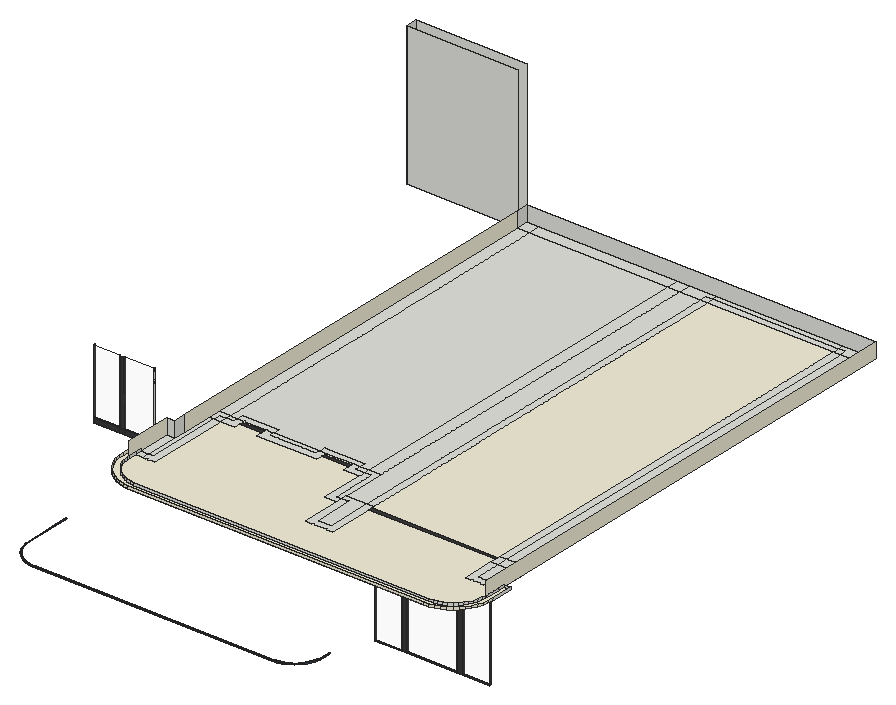
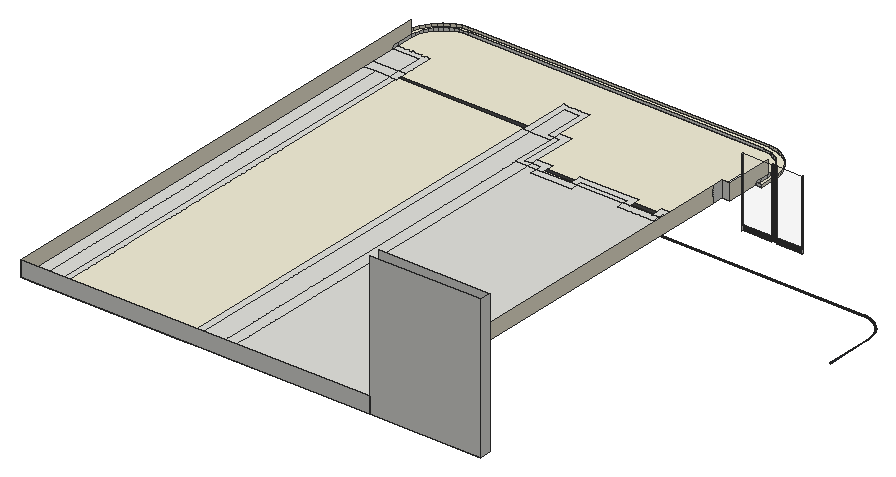
# SketchUp Ruby script. Lengths in inches.
U = 1.inch
M = Sketchup.active_model
def pt(a) = Geom::Point3d.new(a.map { |v| v * U })
def face(e, loops, mat)
  f = e.add_face(loops[0].map { |a| pt(a) })
  loops[1..].each { |l| e.add_face(l.map { |a| pt(a) }).erase! }
  f.material = f.back_material = mat if mat
  f
end
# faces: each face lists its corners as indices into pts; further lists are holes
def faces(e, pts, list, mat = nil) = list.each { |f| face(e, (f[0].is_a?(Array) ? f : [f]).map { |l| l.map { |i| pts[i] } }, mat) }
# xy, xz, yz: faces in a plane at the given z, y or x. An outline is a flat list of corners, or four numbers for a rectangle; further outlines are holes
def ring(l) = l.size == 4 ? [[l[0], l[1]], [l[2], l[1]], [l[2], l[3]], [l[0], l[3]]] : l.each_slice(2).to_a
def flat(e, list, mat, &to3) = list.each { |f| face(e, (f[0].is_a?(Array) ? f : [f]).map { |l| ring(l).map { |u, v| to3.(u, v) } }, mat) }
def xy(e, z, list, mat = nil) = flat(e, list, mat) { |x, y| [x, y, z] }
def xz(e, y, list, mat = nil) = flat(e, list, mat) { |x, z| [x, y, z] }
def yz(e, x, list, mat = nil) = flat(e, list, mat) { |y, z| [x, y, z] }
def lines(e, pts, list) = list.each { |a, b| e.add_line(pt(pts[a]), pt(pts[b])) }
# prism: a flat outline (further loops are holes) pulled along v
def prism(e, loops, v, mat = nil)
  f = face(e, loops, mat); d = Geom::Vector3d.new(v.map { |x| x * U })
  f.pushpull(f.normal.samedirection?(d) ? d.length : -d.length)
end
def box(e, o, s, mat = nil) = prism(e, [[o, [o[0] + s[0], o[1], o[2]], [o[0] + s[0], o[1] + s[1], o[2]], [o[0], o[1] + s[1], o[2]]]], [0, 0, s[2]], mat)
def at(x, y, z, deg = 0) = Geom::Transformation.translation(pt([x, y, z])) * Geom::Transformation.rotation(ORIGIN, Z_AXIS, deg.degrees)
def axes(o, x, y, z) = Geom::Transformation.new([*x, 0, *y, 0, *z, 0, *pt(o).to_a, 1])
def part(name) = M.definitions.add(name)
# library, detail: a bought-in or finely detailed component or shape, given as its bounding box
def library(name, o, s) = part(name).tap { |d| box(d.entities, o, s) }
def detail(e, o, s) = box(e.add_group.entities, o, s)
def put(e, d, t, mat = nil) = e.add_instance(d, t).tap { |i| i.material = mat if mat }
def group(e, t, mat = nil) = e.add_group.tap { |g| g.transformation = t; g.material = mat if mat }.entities
root = M.entities
M.materials.add("0360 AP 9644 Monsoon Midnight-N").color = [56, 67, 95]
M.materials.add("0905 AP 7844 MILD YELLOW").color = [242, 237, 215]
M.materials.add("Glass Clear 001").color = [246, 246, 246]
M.materials["Glass Clear 001"].alpha = 0.1
M.materials.add("[Color M07]").color = [58, 58, 58]
xy(root,164.31,[[267.15,94.4375,287.73,95.4375],[291.07,94.4375,329.62,95.4375],[333.85,94.4375,354.31,95.4375]],"[Color M07]")
xy(root,168,[[57,32.3125,54.18,32.5,51.4,33.05,48.72,33.96,46.1875,35.21,43.84,36.78,41.71,38.65,39.84,40.77,38.27,43.125,37.02,45.66,36.11,48.34,35.56,51.11,35.375,53.9375,35.375,89.9375,35.75,89.9375,35.75,53.9375,35.94,51.16,36.48,48.4375,37.37,45.81,38.6,43.3125,40.14,41,41.98,38.91,44.07,37.08,46.375,35.54,48.87,34.31,51.5,33.41,54.23,32.87,57,32.69,238.5625,32.69,241.34,32.87,244.0625,33.41,246.69,34.31,249.1875,35.54,251.5,37.08,253.59,38.91,255.42,41,256.96,43.3125,258.19,45.81,259.09,48.4375,259.63,51.16,259.81,53.9375,259.81,60.0625,260.1875,60.0625,260.1875,53.9375,260,51.11,259.45,48.34,258.54,45.66,257.29,43.125,255.72,40.77,253.85,38.65,251.73,36.78,249.375,35.21,246.84,33.96,244.16,33.05,241.39,32.5,238.5625,32.3125]])
xy(root,168,[[[57,32.18,54.16,32.36,51.37,32.92,48.67,33.83,46.12,35.09,43.75,36.68,41.61,38.55,39.74,40.69,38.16,43.06,36.9,45.61,35.98,48.31,35.43,51.1,35.24,53.9375,35.24,90.07,35.89,90.07,35.89,53.9375,36.07,51.18,36.61,48.47,37.49,45.86,38.72,43.38,40.25,41.08,42.07,39.01,44.15,37.1875,46.44,35.65,48.92,34.43,51.54,33.54,54.24,33,57,32.82,238.5625,32.82,241.32,33,244.03,33.54,246.64,34.43,249.12,35.65,251.42,37.1875,253.49,39.01,255.3125,41.08,256.85,43.38,258.07,45.86,258.96,48.47,259.5,51.18,259.68,53.9375,259.68,60.2,260.32,60.2,260.32,53.9375,260.14,51.1,259.58,48.31,258.67,45.61,257.41,43.06,255.82,40.69,253.95,38.55,251.81,36.68,249.44,35.09,246.89,33.83,244.19,32.92,241.4,32.36,238.5625,32.18],[57,32.3125,238.5625,32.3125,241.39,32.5,244.16,33.05,246.84,33.96,249.375,35.21,251.73,36.78,253.85,38.65,255.72,40.77,257.29,43.125,258.54,45.66,259.45,48.34,260,51.11,260.1875,53.9375,260.1875,60.0625,259.81,60.0625,259.81,53.9375,259.63,51.16,259.09,48.4375,258.19,45.81,256.96,43.3125,255.42,41,253.59,38.91,251.5,37.08,249.1875,35.54,246.69,34.31,244.0625,33.41,241.34,32.87,238.5625,32.69,57,32.69,54.23,32.87,51.5,33.41,48.87,34.31,46.375,35.54,44.07,37.08,41.98,38.91,40.14,41,38.6,43.3125,37.37,45.81,36.48,48.4375,35.94,51.16,35.75,53.9375,35.75,89.9375,35.375,89.9375,35.375,53.9375,35.56,51.11,36.11,48.34,37.02,45.66,38.27,43.125,39.84,40.77,41.71,38.65,43.84,36.78,46.1875,35.21,48.72,33.96,51.4,33.05,54.18,32.5]]],"0360 AP 9644 Monsoon Midnight-N")
xy(root,168.1875,[[[57,32.18,54.16,32.36,51.37,32.92,48.67,33.83,46.12,35.09,43.75,36.68,41.61,38.55,39.74,40.69,38.16,43.06,36.9,45.61,35.98,48.31,35.43,51.1,35.24,53.9375,35.24,90.07,35.89,90.07,35.89,53.9375,36.07,51.18,36.61,48.47,37.49,45.86,38.72,43.38,40.25,41.08,42.07,39.01,44.15,37.1875,46.44,35.65,48.92,34.43,51.54,33.54,54.24,33,57,32.82,238.5625,32.82,241.32,33,244.03,33.54,246.64,34.43,249.12,35.65,251.42,37.1875,253.49,39.01,255.3125,41.08,256.85,43.38,258.07,45.86,258.96,48.47,259.5,51.18,259.68,53.9375,259.68,60.2,260.32,60.2,260.32,53.9375,260.14,51.1,259.58,48.31,258.67,45.61,257.41,43.06,255.82,40.69,253.95,38.55,251.81,36.68,249.44,35.09,246.89,33.83,244.19,32.92,241.4,32.36,238.5625,32.18],[57,32.3125,238.5625,32.3125,241.39,32.5,244.16,33.05,246.84,33.96,249.375,35.21,251.73,36.78,253.85,38.65,255.72,40.77,257.29,43.125,258.54,45.66,259.45,48.34,260,51.11,260.1875,53.9375,260.1875,60.0625,259.81,60.0625,259.81,53.9375,259.63,51.16,259.09,48.4375,258.19,45.81,256.96,43.3125,255.42,41,253.59,38.91,251.5,37.08,249.1875,35.54,246.69,34.31,244.0625,33.41,241.34,32.87,238.5625,32.69,57,32.69,54.23,32.87,51.5,33.41,48.87,34.31,46.375,35.54,44.07,37.08,41.98,38.91,40.14,41,38.6,43.3125,37.37,45.81,36.48,48.4375,35.94,51.16,35.75,53.9375,35.75,89.9375,35.375,89.9375,35.375,53.9375,35.56,51.11,36.11,48.34,37.02,45.66,38.27,43.125,39.84,40.77,41.71,38.65,43.84,36.78,46.1875,35.21,48.72,33.96,51.4,33.05,54.18,32.5]],[57,32.3125,54.18,32.5,51.4,33.05,48.72,33.96,46.1875,35.21,43.84,36.78,41.71,38.65,39.84,40.77,38.27,43.125,37.02,45.66,36.11,48.34,35.56,51.11,35.375,53.9375,35.375,89.9375,35.75,89.9375,35.75,53.9375,35.94,51.16,36.48,48.4375,37.37,45.81,38.6,43.3125,40.14,41,41.98,38.91,44.07,37.08,46.375,35.54,48.87,34.31,51.5,33.41,54.23,32.87,57,32.69,238.5625,32.69,241.34,32.87,244.0625,33.41,246.69,34.31,249.1875,35.54,251.5,37.08,253.59,38.91,255.42,41,256.96,43.3125,258.19,45.81,259.09,48.4375,259.63,51.16,259.81,53.9375,259.81,60.0625,260.1875,60.0625,260.1875,53.9375,260,51.11,259.45,48.34,258.54,45.66,257.29,43.125,255.72,40.77,253.85,38.65,251.73,36.78,249.375,35.21,246.84,33.96,244.16,33.05,241.39,32.5,238.5625,32.3125]],"0360 AP 9644 Monsoon Midnight-N")
xy(root,168.3125,[[[57,32.18,238.5625,32.18,241.4,32.36,244.19,32.92,246.89,33.83,249.44,35.09,251.81,36.68,253.95,38.55,255.82,40.69,257.41,43.06,258.67,45.61,259.58,48.31,260.14,51.1,260.32,53.9375,260.32,60.2,259.68,60.2,259.68,53.9375,259.5,51.18,258.96,48.47,258.07,45.86,256.85,43.38,255.3125,41.08,253.49,39.01,251.42,37.1875,249.12,35.65,246.64,34.43,244.03,33.54,241.32,33,238.5625,32.82,57,32.82,54.24,33,51.54,33.54,48.92,34.43,46.44,35.65,44.15,37.1875,42.07,39.01,40.25,41.08,38.72,43.38,37.49,45.86,36.61,48.47,36.07,51.18,35.89,53.9375,35.89,90.07,35.24,90.07,35.24,53.9375,35.43,51.1,35.98,48.31,36.9,45.61,38.16,43.06,39.74,40.69,41.61,38.55,43.75,36.68,46.12,35.09,48.67,33.83,51.37,32.92,54.16,32.36],[57,32.3125,54.18,32.5,51.4,33.05,48.72,33.96,46.1875,35.21,43.84,36.78,41.71,38.65,39.84,40.77,38.27,43.125,37.02,45.66,36.11,48.34,35.56,51.11,35.375,53.9375,35.375,89.9375,35.75,89.9375,35.75,53.9375,35.94,51.16,36.48,48.4375,37.37,45.81,38.6,43.3125,40.14,41,41.98,38.91,44.07,37.08,46.375,35.54,48.87,34.31,51.5,33.41,54.23,32.87,57,32.69,238.5625,32.69,241.34,32.87,244.0625,33.41,246.69,34.31,249.1875,35.54,251.5,37.08,253.59,38.91,255.42,41,256.96,43.3125,258.19,45.81,259.09,48.4375,259.63,51.16,259.81,53.9375,259.81,60.0625,260.1875,60.0625,260.1875,53.9375,260,51.11,259.45,48.34,258.54,45.66,257.29,43.125,255.72,40.77,253.85,38.65,251.73,36.78,249.375,35.21,246.84,33.96,244.16,33.05,241.39,32.5,238.5625,32.3125]],[57,32.3125,238.5625,32.3125,241.39,32.5,244.16,33.05,246.84,33.96,249.375,35.21,251.73,36.78,253.85,38.65,255.72,40.77,257.29,43.125,258.54,45.66,259.45,48.34,260,51.11,260.1875,53.9375,260.1875,60.0625,259.81,60.0625,259.81,53.9375,259.63,51.16,259.09,48.4375,258.19,45.81,256.96,43.3125,255.42,41,253.59,38.91,251.5,37.08,249.1875,35.54,246.69,34.31,244.0625,33.41,241.34,32.87,238.5625,32.69,57,32.69,54.23,32.87,51.5,33.41,48.87,34.31,46.375,35.54,44.07,37.08,41.98,38.91,40.14,41,38.6,43.3125,37.37,45.81,36.48,48.4375,35.94,51.16,35.75,53.9375,35.75,89.9375,35.375,89.9375,35.375,53.9375,35.56,51.11,36.11,48.34,37.02,45.66,38.27,43.125,39.84,40.77,41.71,38.65,43.84,36.78,46.1875,35.21,48.72,33.96,51.4,33.05,54.18,32.5]],"0360 AP 9644 Monsoon Midnight-N")
xy(root,231.5,[[160.18,122.9375,192.74,123.43]],"0360 AP 9644 Monsoon Midnight-N")
xy(root,238.39,[[53.24,93.58,73.03,94.27],[76.9,93.58,98.89,94.27]])
xy(root,241.79,[[53.24,93.58,73.03,94.27],[76.86,93.58,98.89,94.27]],"[Color M07]")
xy(root,247.41,[[267.15,94.4375,287.73,95.4375],[291.07,94.4375,329.62,95.4375],[333.85,94.4375,354.31,95.4375]],"[Color M07]")
xy(root,249.32,[[202.6,127.4375,217.88,128.4375]],"[Color M07]")
xy(root,249.81,[[139.74,127.4375,152.36,128.4375]],"[Color M07]")
xy(root,252,[[112.1875,60.0625,112.1875,65.19,117.8125,65.19,117.8125,60.55,116.625,60.55,116.625,60.0625,115.125,60.0625,115.125,60.55,113.3125,60.55,113.3125,60.0625],[118.4375,60.0625,118.4375,60.55,117.8125,60.55,117.8125,65.19,121.68,65.19,121.68,122.9375,126.8125,122.9375,126.8125,60.0625,125.0625,60.0625,125.0625,60.55,123.25,60.55,123.25,60.0625,121.75,60.0625,121.75,60.55,119.9375,60.55,119.9375,60.0625],[241.5625,60.0625,241.5625,95.07,246.69,95.07,246.69,65.19,257.43,65.19,257.43,98.9375,262.5625,98.9375,262.5625,60.0625,257.875,60.0625,257.875,60.55,255.6875,60.55,255.6875,60.0625,253.125,60.0625,253.125,60.55,250.9375,60.55,250.9375,60.0625,248.375,60.0625,248.375,60.55,246.1875,60.55,246.1875,60.0625],[112.1875,65.19,117.8125,89.9375],[117.8125,65.19,121.68,122.9375],
  [246.69,65.19,246.69,95.07,241.5625,95.07,241.5625,98.9375,257.43,98.9375,257.43,65.19],[358.89,65.9375,358.89,89.9375,364.02,89.9375,364.02,71.07,384,71.07,384,65.9375,380.27,65.9375,380.27,66.75,377.92,66.75,377.92,65.9375,375.27,65.9375,375.27,66.75,372.92,66.75,372.92,65.9375,370.27,65.9375,370.27,66.75,367.92,66.75,367.92,65.9375,365.27,65.9375,365.27,66.75,362.92,66.75,362.92,65.9375],[364.02,71.07,384,89.9375],[232.5625,89.9375,232.5625,128.07,237.69,128.07,237.69,95.07,241.5625,95.07,241.5625,89.9375],[358.89,89.9375,364.02,98.9375],
  [364.02,89.9375,384,98.9375],[237.69,95.07,237.69,128.07,232.5625,128.07,232.5625,131.9375,241.5625,131.9375,241.5625,95.07],[241.5625,98.9375,257.43,416.9375],[257.43,98.9375,262.5625,416.9375],[358.89,98.9375,364.02,416.9375],
  [364.02,98.9375,375,416.9375],[375,98.9375,384,425.9375],[117.8125,122.9375,121.68,122.9375,121.68,128.07,126.8125,128.07,126.8125,131.9375,117.8125,131.9375],[121.68,122.9375,126.8125,128.07],[126.8125,122.9375,137.54,122.9375,137.54,131.9375,132.41,131.9375,132.41,128.07,126.8125,128.07],
  [154.56,122.9375,154.56,131.9375,159.6875,131.9375,159.6875,128.07,194.79,128.07,194.79,131.9375,199.92,131.9375,199.92,122.9375],[220.5625,122.9375,220.5625,131.9375,225.69,131.9375,225.69,128.07,232.5625,128.07,232.5625,122.9375],[126.8125,128.07,132.41,131.9375],[159.6875,128.07,194.79,131.9375],[225.69,128.07,232.5625,131.9375],
  [117.8125,131.9375,126.8125,416.9375],[126.8125,131.9375,126.8125,416.9375,232.5625,416.9375,232.5625,131.9375,225.69,131.9375,225.69,137.07,194.79,137.07,194.79,131.9375,159.6875,131.9375,159.6875,137.07,132.41,137.07,132.41,131.9375],[132.41,131.9375,159.6875,137.07],[194.79,131.9375,225.69,137.07],[232.5625,131.9375,241.5625,416.9375],
  [33,416.9375,117.8125,425.9375],[117.8125,416.9375,126.8125,425.9375],[126.8125,416.9375,232.5625,425.9375],[232.5625,416.9375,241.5625,425.9375],[241.5625,416.9375,257.43,416.9375,257.43,422.07,262.5625,422.07,262.5625,425.9375,241.5625,425.9375],
  [257.43,416.9375,262.5625,422.07],[262.5625,416.9375,358.89,422.07],[358.89,416.9375,364.02,422.07],[364.02,416.9375,375,416.9375,375,425.9375,358.89,425.9375,358.89,422.07,364.02,422.07],[262.5625,422.07,358.89,425.9375]])
xy(root,252,[[134.66,24.81,131.02,25.23,127.44,26.12,124.96,27.08,124,27.45,120.76,29.2,117.76,31.35,115.06,33.86,112.69,36.69,110.7,39.8,109.125,43.13,107.98,46.63,107.28,50.26,107.06,53.78,107.06,65.19,112.1875,65.19,112.1875,53.9375,112.38,50.91,112.95,47.92,113.9,45.03,115.2,42.29,116.84,39.73,118.78,37.4,121.01,35.33,123.48,33.56,126.15,32.11,126.8125,31.86,128.99,31.02,131.9375,30.29,134.95,29.9375,360,29.9375,363.13,30.14,366.21,30.76,369.18,31.76,372,33.15,374.61,34.9,376.97,36.97,379.04,39.33,380.78,41.9375,382.17,44.75,383.18,47.73,383.79,50.8,384,53.9375,384,71.07,389.13,71.07,389.13,53.9375,388.88,50.14,388.14,46.4,386.91,42.79,385.23,39.37,383.11,36.2,380.6,33.34,377.73,30.83,374.56,28.71,371.15,27.03,367.54,25.8,363.8,25.06,360,24.81],[134.95,29.9375,131.9375,30.29,128.99,31.02,126.8125,31.86,126.15,32.11,123.48,33.56,121.01,35.33,118.78,37.4,116.84,39.73,115.2,42.29,113.9,45.03,112.95,47.92,112.38,50.91,112.1875,53.9375,112.1875,60.0625,113.3125,60.0625,113.3125,60.55,115.125,60.55,115.125,60.0625,116.625,60.0625,116.625,60.55,118.4375,60.55,118.4375,60.0625,119.9375,60.0625,119.9375,60.55,121.75,60.55,121.75,60.0625,123.25,60.0625,123.25,60.55,125.0625,60.55,125.0625,60.0625,126.8125,60.0625,126.8125,122.9375,137.54,122.9375,137.54,127.4375,154.56,127.4375,154.56,122.9375,199.92,122.9375,199.92,127.4375,220.5625,127.4375,220.5625,122.9375,232.5625,122.9375,232.5625,89.9375,241.5625,89.9375,241.5625,60.0625,246.1875,60.0625,246.1875,60.55,248.375,60.55,248.375,60.0625,250.9375,60.0625,250.9375,60.55,253.125,60.55,253.125,60.0625,255.6875,60.0625,255.6875,60.55,257.875,60.55,257.875,60.0625,262.5625,60.0625,262.5625,94.4375,358.89,94.4375,358.89,65.9375,362.92,65.9375,362.92,66.75,365.27,66.75,365.27,65.9375,367.92,65.9375,367.92,66.75,370.27,66.75,370.27,65.9375,372.92,65.9375,372.92,66.75,375.27,66.75,375.27,65.9375,377.92,65.9375,377.92,66.75,380.27,66.75,380.27,65.9375,384,65.9375,384,53.9375,383.79,50.8,383.18,47.73,382.17,44.75,380.78,41.9375,379.04,39.33,376.97,36.97,374.61,34.9,372,33.15,369.18,31.76,366.21,30.76,363.13,30.14,360,29.9375],[262.5625,96.75,358.89,416.9375],[137.54,130.1875,154.56,131.9375],[199.92,130.1875,220.5625,131.9375]],"0905 AP 7844 MILD YELLOW")
xy(root,252,[[262.5625,94.4375,358.89,96.75],[137.54,127.4375,154.56,130.1875],[199.92,127.4375,220.5625,130.1875]],"[Color M07]")
xz(root,24.81,[[134.66,252,360,253.9375]],"0905 AP 7844 MILD YELLOW")
xz(root,29.9375,[[134.95,252,360,253.9375]])
xz(root,32.18,[[57,168,238.5625,168.1875],[57,168.1875,238.5625,168.3125]],"0360 AP 9644 Monsoon Midnight-N")
xz(root,32.3125,[[57,168,238.5625,168.1875]])
xz(root,32.3125,[[57,168.1875,238.5625,168.3125]],"0360 AP 9644 Monsoon Midnight-N")
xz(root,32.69,[[57,168,238.5625,168.1875]])
xz(root,32.69,[[57,168.1875,238.5625,168.3125]],"0360 AP 9644 Monsoon Midnight-N")
xz(root,32.82,[[57,168,238.5625,168.1875],[57,168.1875,238.5625,168.3125]],"0360 AP 9644 Monsoon Midnight-N")
xz(root,60.0625,[[259.81,168,260.1875,168.1875]])
xz(root,60.0625,[[259.81,168.1875,260.1875,168.3125]],"0360 AP 9644 Monsoon Midnight-N")
xz(root,60.2,[[259.68,168,260.32,168.1875]])
xz(root,60.2,[[259.68,168.1875,260.32,168.3125]],"0360 AP 9644 Monsoon Midnight-N")
xz(root,65.19,[[107.06,252,112.1875,253.9375]])
xz(root,71.07,[[384,252,389.13,253.9375]])
xz(root,89.9375,[[35.375,168,35.75,168.1875],[112.1875,252,117.8125,264]])
xz(root,89.9375,[[35.375,168.1875,35.75,168.3125]],"0360 AP 9644 Monsoon Midnight-N")
xz(root,90.07,[[35.24,168,35.89,168.1875]])
xz(root,90.07,[[35.24,168.1875,35.89,168.3125]],"0360 AP 9644 Monsoon Midnight-N")
xz(root,93.58,[[53.24,238.39,73.03,241.79],[73.03,238.39,76.9,238.39,76.86,241.79,73.03,241.79],[76.9,238.39,98.89,238.39,98.89,241.79,76.86,241.79],[73.03,241.79,76.86,241.79,76.4,291.19,73.03,291.19]],"[Color M07]")
xz(root,94.27,[[53.24,241.79,73.03,291.19],[76.86,241.79,98.89,241.79,98.89,291.19,76.4,291.19]],"Glass Clear 001")
xz(root,94.4375,[[287.73,164.31,291.07,247.41],[329.62,164.31,333.85,247.41]],"[Color M07]")
xz(root,95.4375,[[267.15,164.31,287.73,247.41],[291.07,164.31,329.62,247.41],[333.85,164.31,354.31,247.41]],"Glass Clear 001")
xz(root,416.9375,[[33,252,117.8125,360]])
xz(root,425.9375,[[33,252,117.8125,360],[117.8125,252,384,264]])
yz(root,33,[[416.9375,252,425.9375,360]])
yz(root,35.24,[[53.9375,168,90.07,168.1875],[53.9375,168.1875,90.07,168.3125]],"0360 AP 9644 Monsoon Midnight-N")
yz(root,35.375,[[53.9375,168,89.9375,168.1875]])
yz(root,35.375,[[53.9375,168.1875,89.9375,168.3125]],"0360 AP 9644 Monsoon Midnight-N")
yz(root,35.75,[[53.9375,168,89.9375,168.1875]])
yz(root,35.75,[[53.9375,168.1875,89.9375,168.3125]],"0360 AP 9644 Monsoon Midnight-N")
yz(root,35.89,[[53.9375,168,90.07,168.1875],[53.9375,168.1875,90.07,168.3125]],"0360 AP 9644 Monsoon Midnight-N")
yz(root,53.24,[[93.58,238.39,94.96,241.79],[94.27,241.79,94.96,291.19]])
yz(root,53.24,[[93.58,241.79,94.27,291.19]],"[Color M07]")
yz(root,73.03,[[93.58,241.79,94.27,291.19]],"[Color M07]")
yz(root,98.89,[[93.58,238.39,94.96,241.79],[94.27,241.79,94.96,291.19]])
yz(root,98.89,[[93.58,241.79,94.27,291.19]],"[Color M07]")
yz(root,107.06,[[53.78,252,65.19,253.9375]],"0905 AP 7844 MILD YELLOW")
yz(root,112.1875,[[53.9375,252,60.0625,253.9375],[60.0625,252,65.19,253.9375]])
yz(root,112.1875,[[65.19,252,65.19,253.9375,53.9375,253.9375,53.9375,264,89.9375,264,89.9375,252]],"0905 AP 7844 MILD YELLOW")
yz(root,117.8125,[[89.9375,252,98.79,264],[416.9375,252,425.9375,264]])
yz(root,117.8125,[[98.79,252,416.9375,264]],"0905 AP 7844 MILD YELLOW")
yz(root,259.68,[[53.9375,168,60.2,168.1875],[53.9375,168.1875,60.2,168.3125]],"0360 AP 9644 Monsoon Midnight-N")
yz(root,259.81,[[53.9375,168,60.0625,168.1875]])
yz(root,259.81,[[53.9375,168.1875,60.0625,168.3125]],"0360 AP 9644 Monsoon Midnight-N")
yz(root,260.1875,[[53.9375,168,60.0625,168.1875]])
yz(root,260.1875,[[53.9375,168.1875,60.0625,168.3125]],"0360 AP 9644 Monsoon Midnight-N")
yz(root,260.32,[[53.9375,168,60.2,168.1875],[53.9375,168.1875,60.2,168.3125]],"0360 AP 9644 Monsoon Midnight-N")
yz(root,267.15,[[94.4375,164.31,95.4375,247.41]],"[Color M07]")
yz(root,287.73,[[94.4375,164.31,95.4375,247.41]],"[Color M07]")
yz(root,291.07,[[94.4375,164.31,95.4375,247.41]],"[Color M07]")
yz(root,329.62,[[94.4375,164.31,95.4375,247.41]],"[Color M07]")
yz(root,333.85,[[94.4375,164.31,95.4375,247.41]],"[Color M07]")
yz(root,354.31,[[94.4375,164.31,95.4375,247.41]],"[Color M07]")
yz(root,384,[[53.9375,252,65.9375,253.9375],[65.9375,252,71.07,253.9375]])
yz(root,384,[[71.07,252,425.9375,252,425.9375,264,53.9375,264,53.9375,253.9375,71.07,253.9375]],"0905 AP 7844 MILD YELLOW")
yz(root,389.13,[[53.9375,252,71.07,253.9375]])
p = [[54.16,32.36,168],[57,32.18,168],[57,32.18,168.1875],[54.16,32.36,168.1875],[238.5625,32.18,168],[241.4,32.36,168],
  [241.4,32.36,168.1875],[238.5625,32.18,168.1875],[57,32.3125,168],[54.18,32.5,168],[54.18,32.5,168.1875],[57,32.3125,168.1875],
  [241.39,32.5,168],[238.5625,32.3125,168],[238.5625,32.3125,168.1875],[241.39,32.5,168.1875],[51.37,32.92,168],[51.37,32.92,168.1875],
  [244.19,32.92,168],[244.19,32.92,168.1875],[51.4,33.05,168],[51.4,33.05,168.1875],[244.16,33.05,168],[244.16,33.05,168.1875],
  [54.23,32.87,168],[57,32.69,168],[57,32.69,168.1875],[54.23,32.87,168.1875],[238.5625,32.69,168],[241.34,32.87,168],
  [241.34,32.87,168.1875],[238.5625,32.69,168.1875],[57,32.82,168],[54.24,33,168],[54.24,33,168.1875],[57,32.82,168.1875],
  [241.32,33,168],[238.5625,32.82,168],[238.5625,32.82,168.1875],[241.32,33,168.1875],[48.67,33.83,168],[48.67,33.83,168.1875],
  [51.5,33.41,168],[51.5,33.41,168.1875],[244.0625,33.41,168],[244.0625,33.41,168.1875],[246.89,33.83,168],[246.89,33.83,168.1875],
  [48.72,33.96,168],[48.72,33.96,168.1875],[51.54,33.54,168],[51.54,33.54,168.1875],[244.03,33.54,168],[244.03,33.54,168.1875],
  [246.84,33.96,168],[246.84,33.96,168.1875],[48.87,34.31,168],[48.87,34.31,168.1875],[246.69,34.31,168],[246.69,34.31,168.1875],
  [48.92,34.43,168],[48.92,34.43,168.1875],[246.64,34.43,168],[246.64,34.43,168.1875],[46.12,35.09,168],[46.12,35.09,168.1875],
  [249.44,35.09,168],[249.44,35.09,168.1875],[46.1875,35.21,168],[46.1875,35.21,168.1875],[249.375,35.21,168],[249.375,35.21,168.1875],
  [46.375,35.54,168],[46.375,35.54,168.1875],[249.1875,35.54,168],[249.1875,35.54,168.1875],[46.44,35.65,168],[46.44,35.65,168.1875],
  [249.12,35.65,168],[249.12,35.65,168.1875],[43.75,36.68,168],[43.75,36.68,168.1875],[251.81,36.68,168],[251.81,36.68,168.1875],
  [43.84,36.78,168],[43.84,36.78,168.1875],[251.73,36.78,168],[251.73,36.78,168.1875],[44.07,37.08,168],[44.07,37.08,168.1875],
  [251.5,37.08,168],[251.5,37.08,168.1875],[44.15,37.1875,168],[44.15,37.1875,168.1875],[251.42,37.1875,168],[251.42,37.1875,168.1875],
  [41.61,38.55,168],[41.61,38.55,168.1875],[253.95,38.55,168],[253.95,38.55,168.1875],[41.71,38.65,168],[41.71,38.65,168.1875],
  [253.85,38.65,168],[253.85,38.65,168.1875],[41.98,38.91,168],[41.98,38.91,168.1875],[253.59,38.91,168],[253.59,38.91,168.1875],
  [42.07,39.01,168],[42.07,39.01,168.1875],[253.49,39.01,168],[253.49,39.01,168.1875],[39.74,40.69,168],[39.74,40.69,168.1875],
  [39.84,40.77,168],[39.84,40.77,168.1875],[255.82,40.69,168],[255.82,40.69,168.1875],[255.72,40.77,168],[255.72,40.77,168.1875],
  [40.14,41,168],[40.14,41,168.1875],[255.42,41,168],[255.42,41,168.1875],[40.25,41.08,168],[40.25,41.08,168.1875],
  [255.3125,41.08,168],[255.3125,41.08,168.1875],[38.16,43.06,168],[38.16,43.06,168.1875],[257.41,43.06,168],[257.41,43.06,168.1875],
  [38.27,43.125,168],[38.27,43.125,168.1875],[257.29,43.125,168],[257.29,43.125,168.1875],[38.6,43.3125,168],[38.6,43.3125,168.1875],
  [256.96,43.3125,168],[256.96,43.3125,168.1875],[38.72,43.38,168],[38.72,43.38,168.1875],[256.85,43.38,168],[256.85,43.38,168.1875],
  [36.9,45.61,168],[36.9,45.61,168.1875],[37.02,45.66,168],[37.02,45.66,168.1875],[258.54,45.66,168],[258.54,45.66,168.1875],
  [258.67,45.61,168],[258.67,45.61,168.1875],[37.37,45.81,168],[37.37,45.81,168.1875],[258.19,45.81,168],[258.19,45.81,168.1875],
  [37.49,45.86,168],[37.49,45.86,168.1875],[258.07,45.86,168],[258.07,45.86,168.1875],[35.98,48.31,168],[35.98,48.31,168.1875],
  [259.58,48.31,168],[259.58,48.31,168.1875],[36.11,48.34,168],[36.11,48.34,168.1875],[259.45,48.34,168],[259.45,48.34,168.1875],
  [36.48,48.4375,168],[36.48,48.4375,168.1875],[259.09,48.4375,168],[259.09,48.4375,168.1875],[36.61,48.47,168],[36.61,48.47,168.1875],
  [258.96,48.47,168],[258.96,48.47,168.1875],[35.43,51.1,168],[35.43,51.1,168.1875],[35.56,51.11,168],[35.56,51.11,168.1875],
  [260,51.11,168],[260,51.11,168.1875],[260.14,51.1,168],[260.14,51.1,168.1875],[35.94,51.16,168],[35.94,51.16,168.1875],
  [259.63,51.16,168],[259.63,51.16,168.1875],[36.07,51.18,168],[36.07,51.18,168.1875],[259.5,51.18,168],[259.5,51.18,168.1875],
  [35.24,53.9375,168],[35.24,53.9375,168.1875],[35.375,53.9375,168],[35.375,53.9375,168.1875],[260.1875,53.9375,168],[260.1875,53.9375,168.1875],
  [260.32,53.9375,168],[260.32,53.9375,168.1875],[35.75,53.9375,168],[35.75,53.9375,168.1875],[35.89,53.9375,168],[35.89,53.9375,168.1875],
  [259.68,53.9375,168],[259.68,53.9375,168.1875],[259.81,53.9375,168],[259.81,53.9375,168.1875],[57,32.18,168.3125],[54.16,32.36,168.3125],
  [241.4,32.36,168.3125],[238.5625,32.18,168.3125],[57,32.3125,168.3125],[54.18,32.5,168.3125],[241.39,32.5,168.3125],[238.5625,32.3125,168.3125],
  [51.37,32.92,168.3125],[244.19,32.92,168.3125],[51.4,33.05,168.3125],[244.16,33.05,168.3125],[54.23,32.87,168.3125],[57,32.69,168.3125],
  [238.5625,32.69,168.3125],[241.34,32.87,168.3125],[54.24,33,168.3125],[57,32.82,168.3125],[238.5625,32.82,168.3125],[241.32,33,168.3125],
  [48.67,33.83,168.3125],[51.5,33.41,168.3125],[244.0625,33.41,168.3125],[246.89,33.83,168.3125],[48.72,33.96,168.3125],[51.54,33.54,168.3125],
  [244.03,33.54,168.3125],[246.84,33.96,168.3125],[48.87,34.31,168.3125],[246.69,34.31,168.3125],[48.92,34.43,168.3125],[246.64,34.43,168.3125],
  [46.12,35.09,168.3125],[249.44,35.09,168.3125],[46.1875,35.21,168.3125],[249.375,35.21,168.3125],[46.375,35.54,168.3125],[249.1875,35.54,168.3125],
  [46.44,35.65,168.3125],[249.12,35.65,168.3125],[43.75,36.68,168.3125],[251.81,36.68,168.3125],[43.84,36.78,168.3125],[251.73,36.78,168.3125],
  [44.07,37.08,168.3125],[251.5,37.08,168.3125],[44.15,37.1875,168.3125],[251.42,37.1875,168.3125],[41.61,38.55,168.3125],[253.95,38.55,168.3125],
  [41.71,38.65,168.3125],[253.85,38.65,168.3125],[41.98,38.91,168.3125],[253.59,38.91,168.3125],[42.07,39.01,168.3125],[253.49,39.01,168.3125],
  [39.74,40.69,168.3125],[39.84,40.77,168.3125],[255.72,40.77,168.3125],[255.82,40.69,168.3125],[40.14,41,168.3125],[255.42,41,168.3125],
  [40.25,41.08,168.3125],[255.3125,41.08,168.3125],[38.16,43.06,168.3125],[257.41,43.06,168.3125],[38.27,43.125,168.3125],[257.29,43.125,168.3125],
  [38.6,43.3125,168.3125],[256.96,43.3125,168.3125],[38.72,43.38,168.3125],[256.85,43.38,168.3125],[36.9,45.61,168.3125],[37.02,45.66,168.3125],
  [258.54,45.66,168.3125],[258.67,45.61,168.3125],[37.37,45.81,168.3125],[258.19,45.81,168.3125],[37.49,45.86,168.3125],[258.07,45.86,168.3125],
  [35.98,48.31,168.3125],[259.58,48.31,168.3125],[36.11,48.34,168.3125],[259.45,48.34,168.3125],[36.48,48.4375,168.3125],[259.09,48.4375,168.3125],
  [36.61,48.47,168.3125],[258.96,48.47,168.3125],[35.43,51.1,168.3125],[35.56,51.11,168.3125],[260,51.11,168.3125],[260.14,51.1,168.3125],
  [35.94,51.16,168.3125],[259.63,51.16,168.3125],[36.07,51.18,168.3125],[259.5,51.18,168.3125],[35.24,53.9375,168.3125],[35.375,53.9375,168.3125],
  [260.1875,53.9375,168.3125],[260.32,53.9375,168.3125],[35.75,53.9375,168.3125],[35.89,53.9375,168.3125],[259.68,53.9375,168.3125],[259.81,53.9375,168.3125],
  [76.86,94.27,241.79],[76.4,94.27,291.19],[76.4,93.58,291.19],[76.86,93.58,241.79],[131.02,25.23,252],[134.66,24.81,252],
  [134.66,24.81,253.9375],[131.02,25.23,253.9375],[360,24.81,252],[363.8,25.06,252],[363.8,25.06,253.9375],[360,24.81,253.9375],
  [367.54,25.8,252],[367.54,25.8,253.9375],[127.44,26.12,252],[127.44,26.12,253.9375],[371.15,27.03,252],[371.15,27.03,253.9375],
  [124.96,27.08,252],[124.96,27.08,253.9375],[374.56,28.71,252],[374.56,28.71,253.9375],[124,27.45,252],[124,27.45,253.9375],
  [120.76,29.2,252],[120.76,29.2,253.9375],[377.73,30.83,252],[377.73,30.83,253.9375],[117.76,31.35,252],[117.76,31.35,253.9375],
  [131.9375,30.29,252],[134.95,29.9375,252],[134.95,29.9375,253.9375],[131.9375,30.29,253.9375],[360,29.9375,252],[363.13,30.14,252],
  [363.13,30.14,253.9375],[360,29.9375,253.9375],[366.21,30.76,252],[366.21,30.76,253.9375],[128.99,31.02,252],[128.99,31.02,253.9375],
  [369.18,31.76,252],[369.18,31.76,253.9375],[380.6,33.34,252],[380.6,33.34,253.9375],[126.8125,31.86,252],[126.8125,31.86,253.9375],
  [115.06,33.86,252],[115.06,33.86,253.9375],[372,33.15,252],[372,33.15,253.9375],[126.15,32.11,252],[126.15,32.11,253.9375],
  [123.48,33.56,252],[123.48,33.56,253.9375],[374.61,34.9,252],[374.61,34.9,253.9375],[383.11,36.2,252],[383.11,36.2,253.9375],
  [121.01,35.33,252],[121.01,35.33,253.9375],[112.69,36.69,252],[112.69,36.69,253.9375],[376.97,36.97,252],[376.97,36.97,253.9375],
  [118.78,37.4,252],[118.78,37.4,253.9375],[385.23,39.37,252],[385.23,39.37,253.9375],[110.7,39.8,252],[110.7,39.8,253.9375],
  [379.04,39.33,252],[379.04,39.33,253.9375],[116.84,39.73,252],[116.84,39.73,253.9375],[380.78,41.9375,252],[380.78,41.9375,253.9375],
  [386.91,42.79,252],[386.91,42.79,253.9375],[115.2,42.29,252],[115.2,42.29,253.9375],[109.125,43.13,252],[109.125,43.13,253.9375],
  [382.17,44.75,252],[382.17,44.75,253.9375],[113.9,45.03,252],[113.9,45.03,253.9375],[388.14,46.4,252],[388.14,46.4,253.9375],
  [107.98,46.63,252],[107.98,46.63,253.9375],[383.18,47.73,252],[383.18,47.73,253.9375],[112.95,47.92,252],[112.95,47.92,253.9375],
  [388.88,50.14,252],[388.88,50.14,253.9375],[107.28,50.26,252],[107.28,50.26,253.9375],[383.79,50.8,252],[383.79,50.8,253.9375],
  [112.38,50.91,252],[112.38,50.91,253.9375],[389.13,53.9375,252],[389.13,53.9375,253.9375],[107.06,53.78,252],[107.06,53.78,253.9375],
  [384,53.9375,252],[384,53.9375,253.9375],[112.1875,53.9375,252],[112.1875,53.9375,253.9375]]
faces(root,p,[[0,1,2,3],[4,5,6,7],[16,0,3,17],[5,18,19,6],[32,33,34,35],[36,37,38,39],[40,16,17,41],[18,46,47,19],
  [33,50,51,34],[52,36,39,53],[50,60,61,51],[62,52,53,63],[64,40,41,65],[46,66,67,47],[60,76,77,61],[78,62,63,79],
  [80,64,65,81],[66,82,83,67],[76,92,93,77],[94,78,79,95],[96,80,81,97],[82,98,99,83],[92,108,109,93],[110,94,95,111],
  [112,96,97,113],[98,116,117,99],[108,124,125,109],[126,110,111,127],[128,112,113,129],[116,130,131,117],[124,140,141,125],[142,126,127,143],
  [144,128,129,145],[130,150,151,131],[140,156,157,141],[158,142,143,159],[160,144,145,161],[150,162,163,151],[156,172,173,157],[174,158,159,175],
  [176,160,161,177],[162,182,183,163],[172,188,189,173],[190,174,175,191],[192,176,177,193],[182,198,199,183],[188,202,203,189],[204,190,191,205],
  [3,2,208,209],[7,6,210,211],[10,11,212,213],[14,15,214,215],[17,3,209,216],[6,19,217,210],[21,10,213,218],[15,23,219,214],
  [26,27,220,221],[30,31,222,223],[35,34,224,225],[39,38,226,227],[41,17,216,228],[27,43,229,220],[45,30,223,230],[19,47,231,217],
  [49,21,218,232],[34,51,233,224],[53,39,227,234],[23,55,235,219],[43,57,236,229],[59,45,230,237],[51,61,238,233],[63,53,234,239],
  [65,41,228,240],[47,67,241,231],[69,49,232,242],[55,71,243,235],[57,73,244,236],[75,59,237,245],[61,77,246,238],[79,63,239,247],
  [81,65,240,248],[67,83,249,241],[85,69,242,250],[71,87,251,243],[73,89,252,244],[91,75,245,253],[77,93,254,246],[95,79,247,255],
  [97,81,248,256],[83,99,257,249],[101,85,250,258],[87,103,259,251],[89,105,260,252],[107,91,253,261],[93,109,262,254],[111,95,255,263],
  [113,97,256,264],[115,101,258,265],[103,119,266,259],[99,117,267,257],[105,121,268,260],[123,107,261,269],[109,125,270,262],[127,111,263,271],
  [129,113,264,272],[117,131,273,267],[133,115,265,274],[119,135,275,266],[121,137,276,268],[139,123,269,277],[125,141,278,270],[143,127,271,279],
  [145,129,272,280],[147,133,274,281],[135,149,282,275],[131,151,283,273],[137,153,284,276],[155,139,277,285],[141,157,286,278],[159,143,279,287],
  [161,145,280,288],[151,163,289,283],[165,147,281,290],[149,167,291,282],[153,169,292,284],[171,155,285,293],[157,173,294,286],[175,159,287,295],
  [177,161,288,296],[179,165,290,297],[167,181,298,291],[163,183,299,289],[169,185,300,292],[187,171,293,301],[173,189,302,294],[191,175,295,303],
  [193,177,296,304],[195,179,297,305],[181,197,306,298],[183,199,307,299],[185,201,308,300],[189,203,309,302],[205,191,303,310],[207,187,301,311]],"0360 AP 9644 Monsoon Midnight-N")
faces(root,p,[[8,9,10,11],[12,13,14,15],[9,20,21,10],[22,12,15,23],[24,25,26,27],[28,29,30,31],[42,24,27,43],[29,44,45,30],
  [20,48,49,21],[54,22,23,55],[56,42,43,57],[44,58,59,45],[48,68,69,49],[70,54,55,71],[72,56,57,73],[58,74,75,59],
  [68,84,85,69],[86,70,71,87],[88,72,73,89],[74,90,91,75],[84,100,101,85],[102,86,87,103],[104,88,89,105],[90,106,107,91],
  [100,114,115,101],[118,102,103,119],[120,104,105,121],[106,122,123,107],[114,132,133,115],[134,118,119,135],[136,120,121,137],[122,138,139,123],
  [132,146,147,133],[148,134,135,149],[152,136,137,153],[138,154,155,139],[146,164,165,147],[166,148,149,167],[168,152,153,169],[154,170,171,155],
  [164,178,179,165],[180,166,167,181],[184,168,169,185],[170,186,187,171],[178,194,195,179],[196,180,181,197],[200,184,185,201],[186,206,207,187],
  [342,343,344,345],[346,347,348,349],[347,350,351,348],[352,342,345,353],[350,354,355,351],[358,352,353,359],[354,362,363,355],[364,358,359,365],
  [366,364,365,367],[362,368,369,363],[372,366,367,373],[368,376,377,369],[378,372,373,379],[376,384,385,377],[386,378,379,387],[384,388,389,385],
  [392,386,387,393],[388,396,397,389],[398,392,393,399],[396,404,405,397],[406,398,399,407],[404,412,413,405],[414,406,407,415],[412,420,421,413],
  [422,414,415,423]])
faces(root,p,[[312,313,314,315]],"[Color M07]")
faces(root,p,[[316,317,318,319],[320,321,322,323],[321,324,325,322],[326,316,319,327],[324,328,329,325],[330,326,327,331],[328,332,333,329],[334,330,331,335],
  [336,334,335,337],[332,338,339,333],[340,336,337,341],[338,356,357,339],[360,340,341,361],[356,370,371,357],[374,360,361,375],[370,380,381,371],
  [382,374,375,383],[380,390,391,381],[394,382,383,395],[390,400,401,391],[402,394,395,403],[400,408,409,401],[410,402,403,411],[408,416,417,409],
  [418,410,411,419]],"0905 AP 7844 MILD YELLOW")
